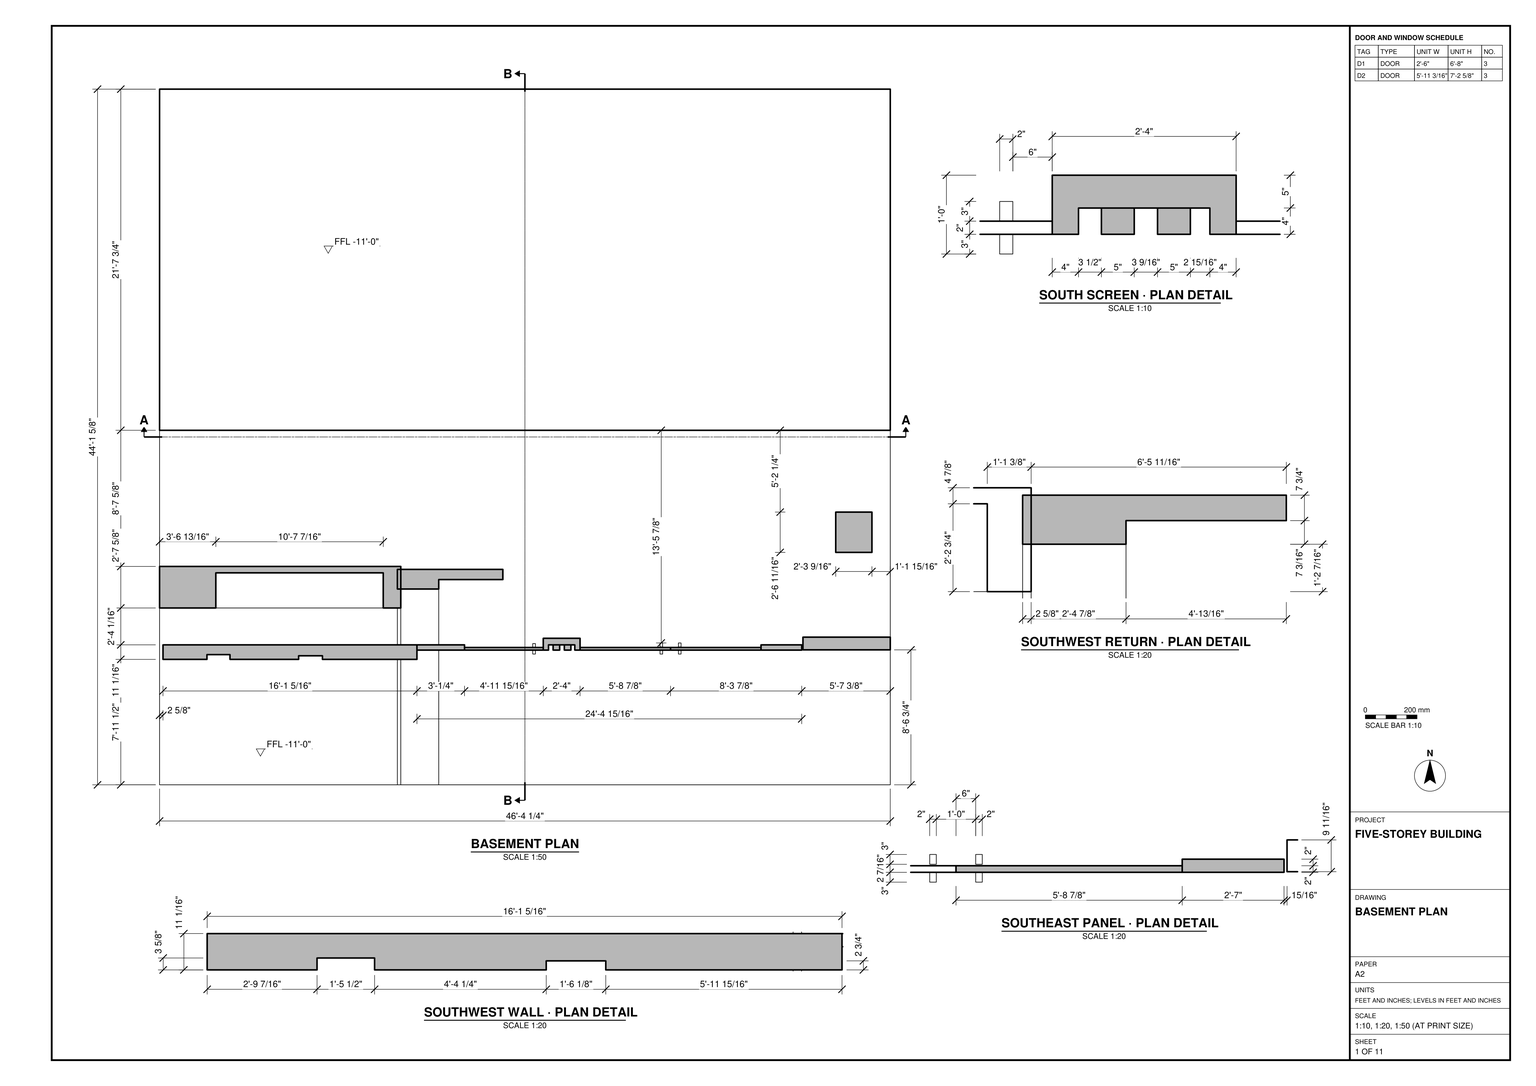
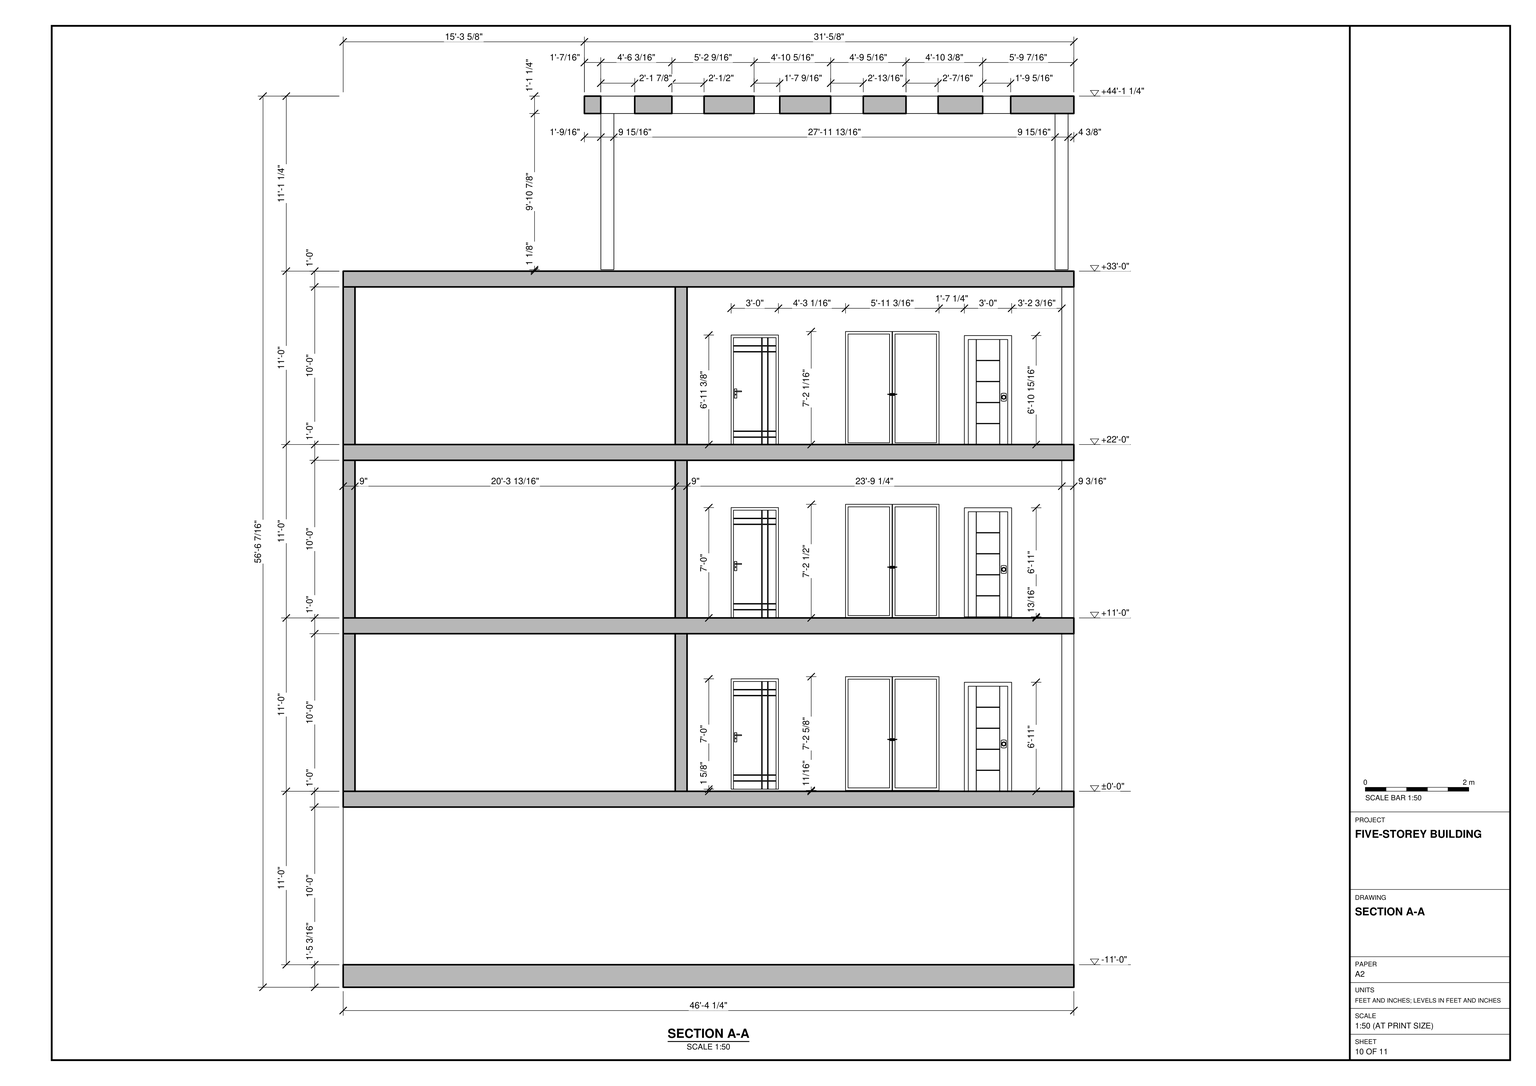
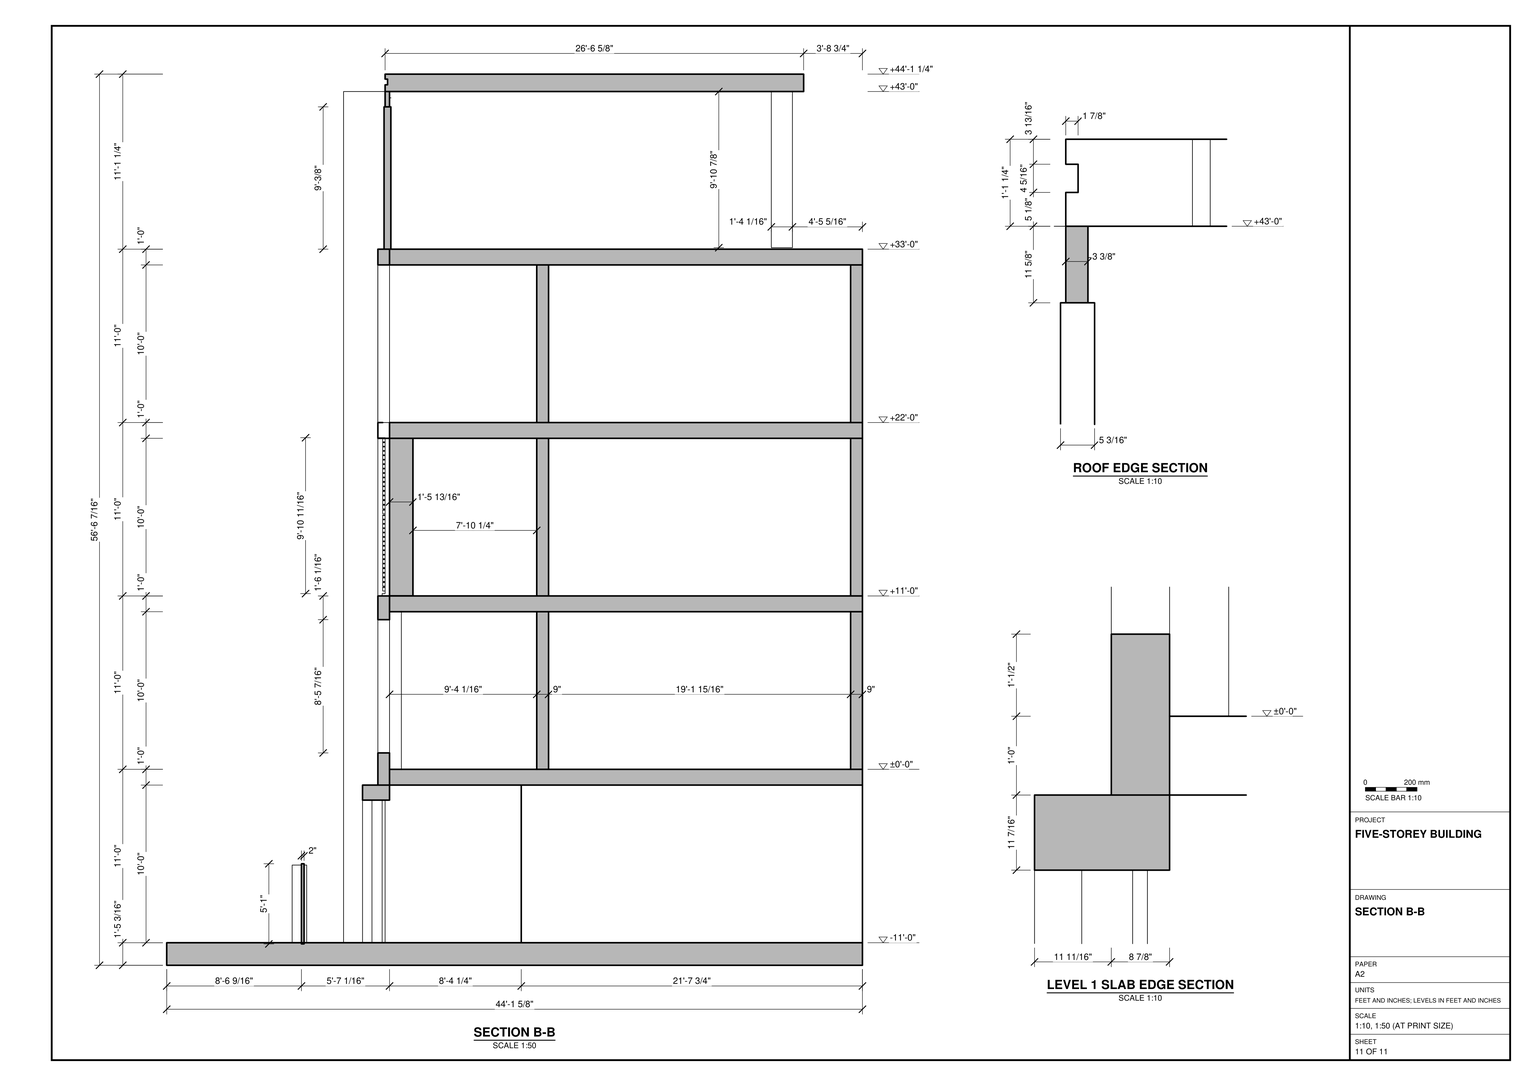
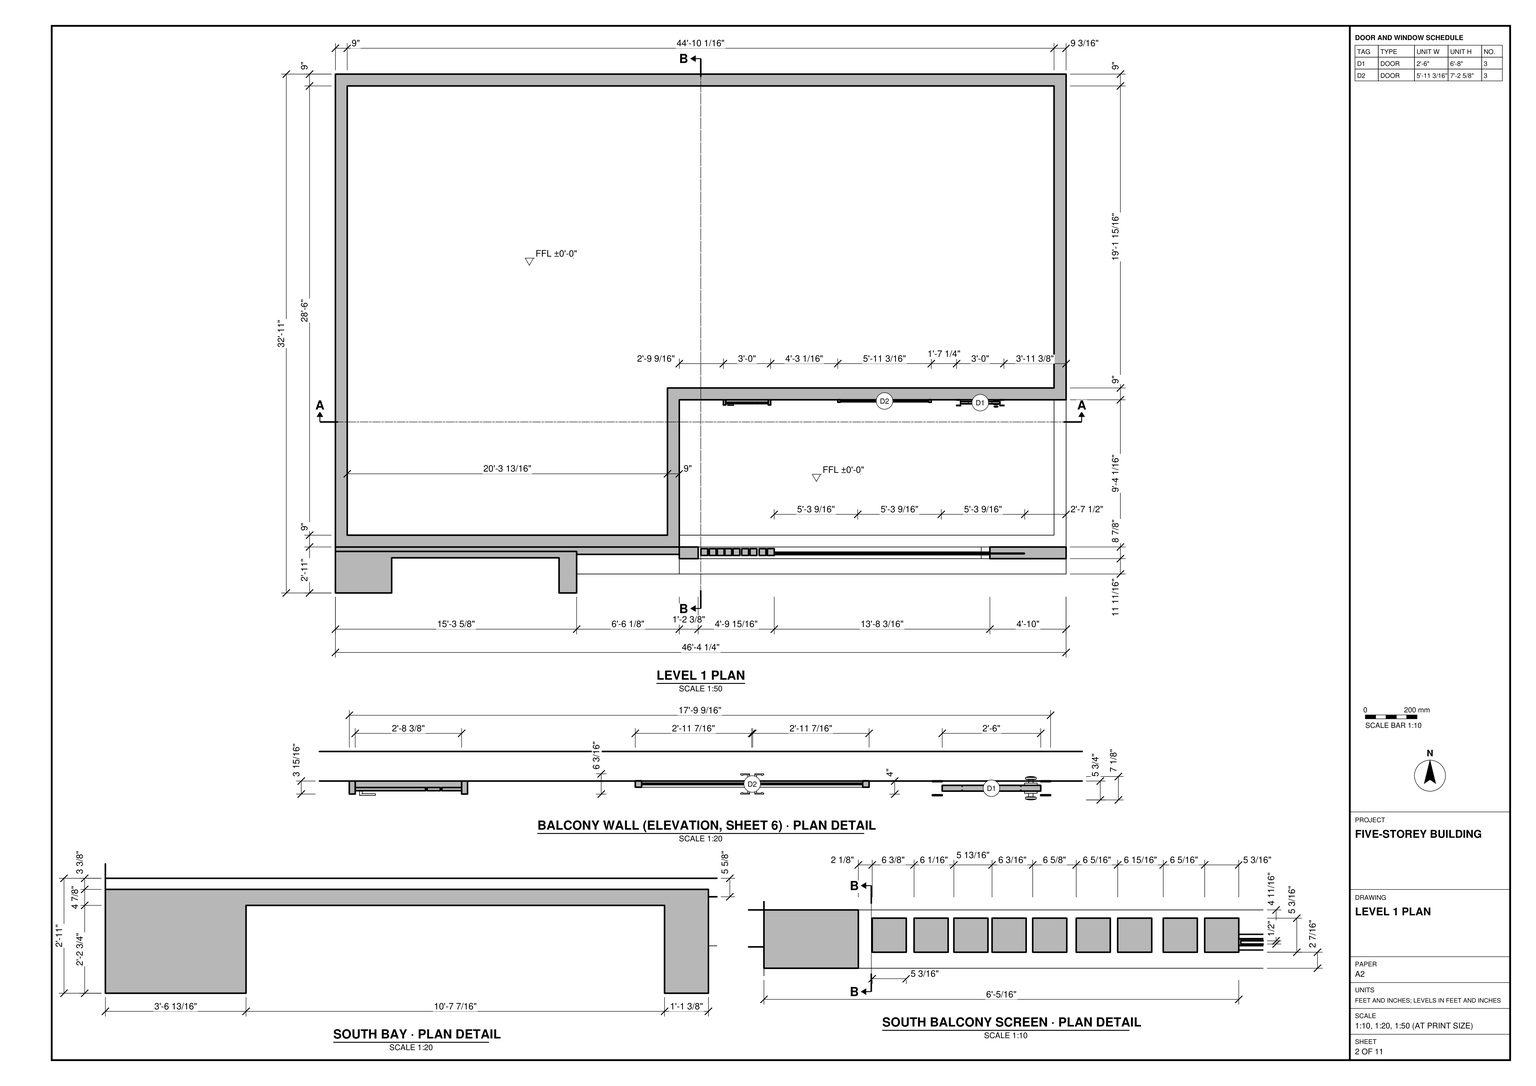
Build the building shown in task_files/diagram_01.pdf in SketchUp. Work in feet and inches. Orient the model with X east–west and Y north–south. The overall extents are 46'-4 1/4" along X, 44'-1 5/8" along Y and 56'-6 7/16" vertically. Set the basement at -11'-0", the ground floor at ±0'-0", and the remaining slab levels at +11'-0", +22'-0" and +33'-0".

Start with the basement slab, which extends south beyond the floors above. Use the enlarged basement plan details to shape the notched southwest wall, its return, the south screen and the southeast panel. Build the stacked floors with the wall thicknesses, slab edges and openings shown in the plans and sections. In section A-A, a pair of doors sits between two single doors; align this arrangement across the three floors shown. Use the plans to locate any stairs, built-in joinery and main furniture shown. Above the top slab, model the canopy supports and roof members, leaving the rest of the slab uncovered. Follow the roof edge section for the stepped profile.

Keep shell elements such as walls, slabs and roof separate as groups or components, and do the same for each furniture or joinery piece. Use components for repeated parts. Any decor and loose items shown may be suitable library components. Save one SketchUp model as output_files/five_storey_building_with_its_partial_rooftop_canopy.skp.

# SketchUp Ruby script. Lengths in inches.
U = 1.inch
M = Sketchup.active_model
def pt(a) = Geom::Point3d.new(a.map { |v| v * U })
def face(e, loops, mat)
  f = e.add_face(loops[0].map { |a| pt(a) })
  loops[1..].each { |l| e.add_face(l.map { |a| pt(a) }).erase! }
  f.material = f.back_material = mat if mat
  f
end
# faces: each face lists its corners as indices into pts; further lists are holes
def faces(e, pts, list, mat = nil) = list.each { |f| face(e, (f[0].is_a?(Array) ? f : [f]).map { |l| l.map { |i| pts[i] } }, mat) }
# xy, xz, yz: faces in a plane at the given z, y or x. An outline is a flat list of corners, or four numbers for a rectangle; further outlines are holes
def ring(l) = l.size == 4 ? [[l[0], l[1]], [l[2], l[1]], [l[2], l[3]], [l[0], l[3]]] : l.each_slice(2).to_a
def flat(e, list, mat, &to3) = list.each { |f| face(e, (f[0].is_a?(Array) ? f : [f]).map { |l| ring(l).map { |u, v| to3.(u, v) } }, mat) }
def xy(e, z, list, mat = nil) = flat(e, list, mat) { |x, y| [x, y, z] }
def xz(e, y, list, mat = nil) = flat(e, list, mat) { |x, z| [x, y, z] }
def yz(e, x, list, mat = nil) = flat(e, list, mat) { |y, z| [x, y, z] }
def lines(e, pts, list) = list.each { |a, b| e.add_line(pt(pts[a]), pt(pts[b])) }
# prism: a flat outline (further loops are holes) pulled along v
def prism(e, loops, v, mat = nil)
  f = face(e, loops, mat); d = Geom::Vector3d.new(v.map { |x| x * U })
  f.pushpull(f.normal.samedirection?(d) ? d.length : -d.length)
end
def box(e, o, s, mat = nil) = prism(e, [[o, [o[0] + s[0], o[1], o[2]], [o[0] + s[0], o[1] + s[1], o[2]], [o[0], o[1] + s[1], o[2]]]], [0, 0, s[2]], mat)
def at(x, y, z, deg = 0) = Geom::Transformation.translation(pt([x, y, z])) * Geom::Transformation.rotation(ORIGIN, Z_AXIS, deg.degrees)
def axes(o, x, y, z) = Geom::Transformation.new([*x, 0, *y, 0, *z, 0, *pt(o).to_a, 1])
def part(name) = M.definitions.add(name)
# library, detail: a bought-in or finely detailed component or shape, given as its bounding box
def library(name, o, s) = part(name).tap { |d| box(d.entities, o, s) }
def detail(e, o, s) = box(e.add_group.entities, o, s)
def put(e, d, t, mat = nil) = e.add_instance(d, t).tap { |i| i.material = mat if mat }
def group(e, t, mat = nil) = e.add_group.tap { |g| g.transformation = t; g.material = mat if mat }.entities
root = M.entities
M.materials.add("Glass_Window_Neutral\#2").color = [0, 0, 0]
M.materials["Glass_Window_Neutral\#2"].alpha = 0.125
M.materials.add("Iron_Blurry_5cm").color = [3, 3, 3]
M.materials.add("Material5, met").color = [196, 146, 107]
M.materials.add("[Color M00]").color = [255, 255, 255]
M.materials.add("[Color M09]").color = [0, 0, 0]
M.materials.add("[Granite Brown]").color = [126, 104, 91]
M.materials.add("[Granite Dark Gray]").color = [69, 68, 68]
M.materials.add("[Grass Dark Green]").color = [106, 157, 55]
M.materials.add("[Polished Concrete New]").color = [200, 200, 203]
M.materials.add("[Sandstone]").color = [118, 81, 52]
M.materials.add("[Stone Marble]").color = [214, 206, 203]
M.materials.add("[Translucent Glass Blue]").color = [100, 149, 237]
M.materials["[Translucent Glass Blue]"].alpha = 0.5
M.materials.add("polished steel").color = [183, 187, 190]
M.materials.add("polished, Blacktop Old 01").color = [132, 136, 139]
M.materials.add("steel").color = [179, 179, 179]
c1 = library("glass door",[0,0,0],[6.2,71.19,86.61])
c2 = library("Untitled (14)",[0,0,0],[7.13,36,83])
c3 = library("Untitled",[0,0,0],[36,4.39,84])
c4 = part("Framed glazing panel")
g1 = group(c4.entities,at(0,26.17,94.49),"[Color M09]")
xy(g1,-94.49,[[0,-26.17,1.18,0]],"Iron_Blurry_5cm")
xy(g1,-93.8,[[0,-25.51,0.59,-0.67],[0.59,-25.51,1.18,-0.67]],"Iron_Blurry_5cm")
xy(g1,-70.52,[[0.59,-25.51,1.18,-0.67]],"Iron_Blurry_5cm")
xy(g1,-69.84,[[0.59,-25.51,1.18,-0.67]],"Iron_Blurry_5cm")
xy(g1,-47.24,[[0.59,-25.51,1.18,-0.67]],"Iron_Blurry_5cm")
xy(g1,-46.56,[[0.59,-25.51,1.18,-0.67]],"Iron_Blurry_5cm")
xy(g1,-23.97,[[0.59,-25.51,1.18,-0.67]],"Iron_Blurry_5cm")
xy(g1,-23.28,[[0.59,-25.51,1.18,-0.67]],"Iron_Blurry_5cm")
xy(g1,-0.6875,[[0,-25.51,0.59,-0.67],[0.59,-25.51,1.18,-0.67]],"Iron_Blurry_5cm")
xy(g1,0,[[0,-26.17,1.18,0]],"Iron_Blurry_5cm")
xz(g1,-26.17,[[0,-94.49,1.18,0]],"Iron_Blurry_5cm")
xz(g1,-25.51,[[0,-93.8,0.59,-0.6875],[0.59,-93.8,1.18,-70.52],[0.59,-70.52,1.18,-69.84],[0.59,-69.84,1.18,-47.24],[0.59,-47.24,1.18,-46.56],
  [0.59,-46.56,1.18,-23.97],[0.59,-23.97,1.18,-23.28],[0.59,-23.28,1.18,-0.6875]],"Iron_Blurry_5cm")
xz(g1,-0.67,[[0,-93.8,0.59,-0.6875],[0.59,-93.8,1.18,-70.52],[0.59,-70.52,1.18,-69.84],[0.59,-69.84,1.18,-47.24],[0.59,-47.24,1.18,-46.56],
  [0.59,-46.56,1.18,-23.97],[0.59,-23.97,1.18,-23.28],[0.59,-23.28,1.18,-0.6875]],"Iron_Blurry_5cm")
xz(g1,0,[[0,-94.49,1.18,0]],"Iron_Blurry_5cm")
yz(g1,0,[[[-26.17,-94.49,0,0],[-25.51,-93.8,-0.67,-0.6875]]],"Iron_Blurry_5cm")
yz(g1,0.59,[[-25.51,-93.8,-0.67,-70.52],[-25.51,-69.84,-0.67,-47.24],[-25.51,-46.56,-0.67,-23.97],[-25.51,-23.28,-0.67,-0.6875]],"Glass_Window_Neutral\#2")
yz(g1,0.59,[[-25.51,-70.52,-0.67,-69.84],[-25.51,-47.24,-0.67,-46.56],[-25.51,-23.97,-0.67,-23.28]],"Iron_Blurry_5cm")
yz(g1,1.18,[[[-26.17,-94.49,0,0],[-25.51,-93.8,-0.67,-0.6875]],[-25.51,-70.52,-0.67,-69.84],[-25.51,-47.24,-0.67,-46.56],[-25.51,-23.97,-0.67,-23.28]],"Iron_Blurry_5cm")
g2 = group(c4.entities,at(0,52.35,94.49),"[Color M09]")
xy(g2,-94.49,[[0,-26.17,1.18,0]],"Iron_Blurry_5cm")
xy(g2,-93.8,[[0,-25.51,0.59,-0.67],[0.59,-25.51,1.18,-0.67]],"Iron_Blurry_5cm")
xy(g2,-70.52,[[0.59,-25.51,1.18,-0.67]],"Iron_Blurry_5cm")
xy(g2,-69.84,[[0.59,-25.51,1.18,-0.67]],"Iron_Blurry_5cm")
xy(g2,-47.24,[[0.59,-25.51,1.18,-0.67]],"Iron_Blurry_5cm")
xy(g2,-46.56,[[0.59,-25.51,1.18,-0.67]],"Iron_Blurry_5cm")
xy(g2,-23.97,[[0.59,-25.51,1.18,-0.67]],"Iron_Blurry_5cm")
xy(g2,-23.28,[[0.59,-25.51,1.18,-0.67]],"Iron_Blurry_5cm")
xy(g2,-0.6875,[[0,-25.51,0.59,-0.67],[0.59,-25.51,1.18,-0.67]],"Iron_Blurry_5cm")
xy(g2,0,[[0,-26.17,1.18,0]],"Iron_Blurry_5cm")
xz(g2,-26.17,[[0,-94.49,1.18,0]],"Iron_Blurry_5cm")
xz(g2,-25.51,[[0,-93.8,0.59,-0.6875],[0.59,-93.8,1.18,-70.52],[0.59,-70.52,1.18,-69.84],[0.59,-69.84,1.18,-47.24],[0.59,-47.24,1.18,-46.56],
  [0.59,-46.56,1.18,-23.97],[0.59,-23.97,1.18,-23.28],[0.59,-23.28,1.18,-0.6875]],"Iron_Blurry_5cm")
xz(g2,-0.67,[[0,-93.8,0.59,-0.6875],[0.59,-93.8,1.18,-70.52],[0.59,-70.52,1.18,-69.84],[0.59,-69.84,1.18,-47.24],[0.59,-47.24,1.18,-46.56],
  [0.59,-46.56,1.18,-23.97],[0.59,-23.97,1.18,-23.28],[0.59,-23.28,1.18,-0.6875]],"Iron_Blurry_5cm")
xz(g2,0,[[0,-94.49,1.18,0]],"Iron_Blurry_5cm")
yz(g2,0,[[[-26.17,-94.49,0,0],[-25.51,-93.8,-0.67,-0.6875]]],"Iron_Blurry_5cm")
yz(g2,0.59,[[-25.51,-93.8,-0.67,-70.52],[-25.51,-69.84,-0.67,-47.24],[-25.51,-46.56,-0.67,-23.97],[-25.51,-23.28,-0.67,-0.6875]],"Glass_Window_Neutral\#2")
yz(g2,0.59,[[-25.51,-70.52,-0.67,-69.84],[-25.51,-47.24,-0.67,-46.56],[-25.51,-23.97,-0.67,-23.28]],"Iron_Blurry_5cm")
yz(g2,1.18,[[[-26.17,-94.49,0,0],[-25.51,-93.8,-0.67,-0.6875]],[-25.51,-70.52,-0.67,-69.84],[-25.51,-47.24,-0.67,-46.56],[-25.51,-23.97,-0.67,-23.28]],"Iron_Blurry_5cm")
c5 = library("Wagner Glass Railing",[9.08,102.375,1.53],[2.51,145.5,42.05])
c6 = part("faewg")
xy(c6.entities,0,[[0,-3,2,0]])
xy(c6.entities,1,[[0,-2,2,0]])
xy(c6.entities,23,[[0,-2,2,0]])
xy(c6.entities,24,[[0,-3,2,0]])
xz(c6.entities,-3,[[0,0,2,24]],"polished steel")
xz(c6.entities,-2,[[0,1,2,23]])
xz(c6.entities,0,[[0,0,2,1],[0,23,2,24]])
yz(c6.entities,0,[[-3,0,-3,24,0,24,0,23,-2,23,-2,1,0,1,0,0]])
yz(c6.entities,2,[[-3,0,0,0,0,1,-2,1,-2,23,0,23,0,24,-3,24]])
c7 = part("reg")
xy(c7.entities,0,[[-8.95,3,59.93,5]])
xy(c7.entities,18,[[51.93,0,53.93,3]],"steel")
xy(c7.entities,19,[[51.93,1,53.93,3]],"steel")
xy(c7.entities,41,[[51.93,1,53.93,3]],"steel")
xy(c7.entities,42,[[51.93,0,53.93,3]],"steel")
xy(c7.entities,61,[[-8.95,3,59.93,5]])
xz(c7.entities,0,[[51.93,18,53.93,42]],"polished steel")
xz(c7.entities,1,[[51.93,19,53.93,41]],"steel")
xz(c7.entities,3,[[[-8.95,0,59.93,61],[51.93,18,53.93,19],[51.93,41,53.93,42]]])
xz(c7.entities,3,[[51.93,18,53.93,19],[51.93,41,53.93,42]],"steel")
xz(c7.entities,5,[[-8.95,0,59.93,61]])
yz(c7.entities,-8.95,[[3,0,5,61]])
yz(c7.entities,51.93,[[0,18,0,42,3,42,3,41,1,41,1,19,3,19,3,18]],"steel")
yz(c7.entities,53.93,[[0,18,3,18,3,19,1,19,1,41,3,41,3,42,0,42]],"steel")
yz(c7.entities,59.93,[[3,0,5,61]])
put(c7.entities,c6,axes([51.93,5.4375,42],[1,0,0],[0,-1,0],[0,0,-1]),"steel")
c8 = part("e3f")
xy(c8.entities,0,[[0,-2,59.93,0]])
xy(c8.entities,18,[[51.93,-5,53.93,-2]],"steel")
xy(c8.entities,19,[[51.93,-4,53.93,-2]],"steel")
xy(c8.entities,41,[[51.93,-4,53.93,-2]],"steel")
xy(c8.entities,42,[[51.93,-5,53.93,-2]],"steel")
xy(c8.entities,61,[[0,-2,59.93,0]])
xz(c8.entities,-5,[[51.93,18,53.93,42]],"polished steel")
xz(c8.entities,-4,[[51.93,19,53.93,41]],"steel")
xz(c8.entities,-2,[[[0,0,59.93,61],[51.93,41,53.93,42],[51.93,18,53.93,19]]])
xz(c8.entities,-2,[[51.93,18,53.93,19],[51.93,41,53.93,42]],"steel")
xz(c8.entities,0,[[0,0,59.93,61]])
yz(c8.entities,0,[[-2,0,0,61]])
yz(c8.entities,51.93,[[-5,18,-5,42,-2,42,-2,41,-4,41,-4,19,-2,19,-2,18]],"steel")
yz(c8.entities,53.93,[[-5,18,-2,18,-2,19,-4,19,-4,41,-2,41,-2,42,-5,42]],"steel")
yz(c8.entities,59.93,[[-2,0,0,61]])
put(c8.entities,c6,axes([51.93,0,42],[1,0,0],[0,-1,0],[0,0,-1]),"steel")
c9 = part("gbsrtn")
put(c9.entities,c7,at(402.95,-3,0))
put(c9.entities,c8,at(306.07,2,0))
put(c9.entities,c7,axes([522.82,-3,0],[-1,0,0],[0,1,0],[0,0,1]))
g3 = group(c9.entities,at(366,9,0),"polished, Blacktop Old 01")
xy(g3,0,[[0,-9,0,0,28,0,28,-9,24,-9,24,-5,4,-5,4,-9]])
xy(g3,60,[[0,-9,4,-9,4,-5,24,-5,24,-9,28,-9,28,0,0,0]],"[Polished Concrete New]")
xz(g3,-9,[[0,0,4,60],[24,0,28,60]],"[Polished Concrete New]")
xz(g3,-5,[[4,0,24,60]],"Material5, met")
xz(g3,0,[[0,0,28,60]])
yz(g3,0,[[-9,0,0,60]],"[Polished Concrete New]")
yz(g3,4,[[-9,0,-5,60]],"polished, Blacktop Old 01")
yz(g3,24,[[-9,0,-5,60]],"polished, Blacktop Old 01")
yz(g3,28,[[-9,0,0,60]],"[Polished Concrete New]")
g4 = group(c9.entities,at(12.5,0,0))
prism(g4,[[[365.99,4,0],[365.99,4,4],[365.99,4,56],[365.99,4,60],[365.99,0,60],[365.99,0,0]]],[-5,0,0])
prism(g4,[[[374.53,4,0],[374.53,4,4],[374.53,4,56],[374.53,4,60],[374.53,0,60],[374.53,0,0]]],[-5,0,0])
g5 = group(c9.entities,at(29.55,0,0))
box(g5,[502.22,0,0],[31,4,60],"[Polished Concrete New]")
box(g5,[240.29,0,0],[36.23,4,60],"[Polished Concrete New]")
c10 = part("main gate")
put(c10.entities,c9,at(-149.07,478.25,-161.76),"[Grass Dark Green]")
c11 = part("Group\#1")
box(c11.entities,[0,-360,0],[556.25,360,12])
c12 = part("Group\#9")
box(c12.entities,[0,0,0],[5.1875,5.1875,132])
c13 = part("Group\#3")
box(c13.entities,[0,0,0],[5.1875,5.1875,101.4375])
c14 = part("Group\#5")
box(c14.entities,[0,0,0],[5.0625,5.0625,87.3125])
c15 = part("Group\#7")
prism(c15.entities,[[[0,0,0],[0,0,3.13],[78.15,0,3.13],[78.15,0,2.68],[78.15,0,0]]],[0,-1.8125,0])
prism(c15.entities,[[[0,0,-3.3125],[0,0,-0.18],[78.15,0,-0.18],[78.15,0,-0.64],[78.15,0,-3.3125]]],[0,-1.8125,0])
prism(c15.entities,[[[0,-1.8125,-3.49],[0,-1.8125,-6.625],[78.15,-1.8125,-6.625],[78.15,-1.8125,-3.95],[78.15,-1.8125,-3.49]]],[0,1.8125,0])
prism(c15.entities,[[[0,0,-9.875],[0,0,-6.74],[78.15,0,-6.74],[78.15,0,-7.2],[78.15,0,-9.875]]],[0,-1.8125,0])
prism(c15.entities,[[[0,0,-13.25],[0,0,-10.12],[78.15,0,-10.12],[78.15,0,-10.57],[78.15,0,-13.25]]],[0,-1.8125,0])
prism(c15.entities,[[[0,-1.8125,-13.49],[0,-1.8125,-16.625],[78.15,-1.8125,-16.625],[78.15,-1.8125,-13.95],[78.15,-1.8125,-13.49]]],[0,1.8125,0])
prism(c15.entities,[[[0,0,-20],[0,0,-16.87],[78.15,0,-16.87],[78.15,0,-17.32],[78.15,0,-20]]],[0,-1.8125,0])
prism(c15.entities,[[[0,0,-23.375],[0,0,-20.24],[78.15,0,-20.24],[78.15,0,-20.7],[78.15,0,-23.375]]],[0,-1.8125,0])
prism(c15.entities,[[[0,-1.8125,-23.62],[0,-1.8125,-26.75],[78.15,-1.8125,-26.75],[78.15,-1.8125,-24.07],[78.15,-1.8125,-23.62]]],[0,1.8125,0])
prism(c15.entities,[[[0,0,-30.125],[0,0,-26.99],[78.15,0,-26.99],[78.15,0,-27.45],[78.15,0,-30.125]]],[0,-1.8125,0])
prism(c15.entities,[[[0,-1.8125,-30.43],[0,-1.8125,-33.5625],[78.15,-1.8125,-33.5625],[78.15,-1.8125,-30.89],[78.15,-1.8125,-30.43]]],[0,1.8125,0])
prism(c15.entities,[[[0,-1.8125,-33.74],[0,-1.8125,-36.875],[78.15,-1.8125,-36.875],[78.15,-1.8125,-34.2],[78.15,-1.8125,-33.74]]],[0,1.8125,0])
prism(c15.entities,[[[0,-1.8125,-37.31],[0,-1.8125,-40.4375],[78.15,-1.8125,-40.4375],[78.15,-1.8125,-37.76],[78.15,-1.8125,-37.31]]],[0,1.8125,0])
prism(c15.entities,[[[0,-1.8125,-40.74],[0,-1.8125,-43.875],[78.15,-1.8125,-43.875],[78.15,-1.8125,-41.2],[78.15,-1.8125,-40.74]]],[0,1.8125,0])
prism(c15.entities,[[[0,-1.8125,-44.37],[0,-1.8125,-47.5],[78.15,-1.8125,-47.5],[78.15,-1.8125,-44.82],[78.15,-1.8125,-44.37]]],[0,1.8125,0])
prism(c15.entities,[[[0,-1.8125,-47.87],[0,-1.8125,-51],[78.15,-1.8125,-51],[78.15,-1.8125,-48.32],[78.15,-1.8125,-47.87]]],[0,1.8125,0])
prism(c15.entities,[[[0,0,-54.75],[0,0,-51.62],[78.15,0,-51.62],[78.15,0,-52.07],[78.15,0,-54.75]]],[0,-1.8125,0])
c16 = part("Group\#8")
box(c16.entities,[0,-0.6875,0],[69.3,0.6875,3.73])
c17 = part("Group\#4")
box(c17.entities,[0,0,0],[5.1875,5.1875,108.35])
c18 = part("Group\#10")
box(c18.entities,[0,0,0],[9.9375,16.08,118.875])
xy(root,-149.1875,[[0,0,556.25,529.625]])
xy(root,-132,[[0,0,181.03,0,181.03,95.49,124,95.49,124,98.24,105.86,98.24,105.86,95.49,53.6,95.49,53.6,99.12,36.07,99.12,36.07,95.49,2.61,95.49,2.61,106.55,181.03,106.55,181.03,134.625,0,134.625],[212.51,0,556.25,0,556.25,102.74,489.78,102.74,489.78,112.42,556.25,112.42,556.25,269.9,0,269.9,0,166.25,183.63,166.25,183.63,164,261.33,164,261.33,156.25,212.51,156.25],[181.03,0,183.63,95.49],[183.63,0,212.51,0,212.51,149.0625,183.63,149.0625,183.63,106.55,195.93,106.55,195.93,95.49,183.63,95.49],[181.03,106.55,183.63,134.625],
  [0,134.625,0,166.25,183.63,166.25,183.63,164,181.03,164,181.03,134.625],[181.03,134.625,183.63,149.0625],[181.03,149.0625,183.63,164],[183.63,149.0625,212.51,164],[212.51,156.25,261.33,164],
  [212.51,156.25,261.33,164],[0,269.9,556.25,529.625]])
xy(root,-117.02,[[42.83,134.625,170.27,161.375]])
xy(root,-72.89,[[2.61,95.49,36.07,95.49,36.07,99.12,53.6,99.12,53.6,95.49,105.86,95.49,105.86,98.24,124,98.24,124,95.49,195.93,95.49,195.93,106.55,2.61,106.55],[489.78,102.74,556.25,112.42]])
xy(root,-23.4375,[[212.51,149.0625,212.51,156.25,261.33,156.25,261.33,164,261.78,164,261.78,169.625,556.25,169.625,556.25,149.0625]])
xy(root,-12,[[181.03,149.0625,261.78,164],[261.78,149.0625,556.25,160.75],[261.78,160.75,556.25,169.625],[183.63,164,183.63,166.25,0,166.25,0,169.625,261.78,169.625,261.78,164],[0,269.9,556.25,529.625]])
xy(root,0,[[[0,169.625,261.78,169.625,261.78,281.6875,556.25,281.6875,556.25,529.625,0,529.625],[9,178.625,9,520.625,547.0625,520.625,547.0625,290.6875,252.78,290.6875,252.78,178.625]],[261.78,169.625,556.25,169.625,556.25,281.6875,547.0625,281.6875,547.0625,178.625,261.78,178.625],[9,178.625,252.78,178.625,252.78,290.6875,547.0625,290.6875,547.0625,520.625,9,520.625]])
xy(root,0,[[261.78,178.625,547.0625,281.6875]],"[Color M00]")
xy(root,12.5,[[276.15,160.75,491.63,169.625]])
xy(root,74.73,[[74.54,149.875,144.61,161.375]],"[Stone Marble]")
xy(root,82.84,[[82.66,149.875,136.49,161.375]],"[Stone Marble]")
xy(root,113.9375,[[276.15,160.75,488.01,169.625],[488.01,160.75,498.24,169.625]])
xy(root,120,[[[0,169.625,261.78,169.625,261.78,281.6875,556.25,281.6875,556.25,529.625,0,529.625],[9,178.625,9,520.625,547.0625,520.625,547.0625,290.6875,252.78,290.6875,252.78,178.625]]])
xy(root,132,[[261.78,160.75,556.25,169.625],[[0,169.625,261.78,169.625,261.78,281.6875,556.25,281.6875,556.25,529.625,0,529.625],[9,178.625,9,520.625,547.0625,520.625,547.0625,290.6875,252.78,290.6875,252.78,178.625]],[261.78,169.625,556.25,169.625,556.25,281.6875,547.0625,281.6875,547.0625,178.625,261.78,178.625],[9,178.625,252.78,178.625,252.78,290.6875,547.0625,290.6875,547.0625,520.625,9,520.625]])
xy(root,132.0625,[[519.2,160.75,556.25,170.3125],[261.78,169.625,261.78,187.4375,556.25,187.4375,556.25,170.3125,519.2,170.3125,519.2,169.625]])
xy(root,133.78,[[183.63,164,261.78,166.25]])
xy(root,152.84,[[329.09,169.625,500.01,187.4375]])
xy(root,234.78,[[329.91,169.625,500.01,187.4375]])
xy(root,252,[[261.78,160.75,519.2,169.625],[519.2,160.75,556.25,169.625],[[0,169.625,261.78,169.625,261.78,281.6875,556.25,281.6875,556.25,529.625,0,529.625],[9,178.625,9,520.625,547.0625,520.625,547.0625,290.6875,252.78,290.6875,252.78,178.625]],[519.2,169.625,556.25,170.3125]])
xy(root,252.46,[[183.63,160.6875,261.78,166.25]],"[Granite Dark Gray]")
xy(root,264,[[276.15,160.75,481.8,160.75,481.8,169.625,283.3125,169.625,283.3125,164.4375,278.125,164.4375,278.125,169.625,276.15,169.625],[[0,169.625,261.78,169.625,261.78,281.6875,556.25,281.6875,556.25,529.625,0,529.625],[9,178.625,9,520.625,547.0625,520.625,547.0625,290.6875,252.78,290.6875,252.78,178.625]],[481.8,169.625,498.24,169.9375],[9,178.625,252.78,178.625,252.78,290.6875,547.0625,290.6875,547.0625,520.625,9,520.625]])
xy(root,384,[[276.15,160.75,477.47,169.625],[[0,169.625,261.78,169.625,261.78,281.6875,556.25,281.6875,556.25,529.625,0,529.625],[9,178.625,9,520.625,547.0625,520.625,547.0625,290.6875,252.78,290.6875,252.78,178.625]]])
xy(root,388.11,[[82.66,149.875,136.49,161.375]],"[Stone Marble]")
xy(root,396,[[261.78,160.75,556.25,169.625],[0,166.25,183.63,169.625]])
xy(root,396,[[183.63,160.6875,192.48,166.25],[192.48,160.6875,261.78,167.9375]],"[Granite Dark Gray]")
xy(root,396.23,[[74.54,149.875,144.61,161.375]],"[Stone Marble]")
xy(root,497.48,[[42.83,134.625,170.27,161.375]])
xy(root,504.35,[[192.48,166.25,192.48,167.9375,261.78,167.9375,261.78,169.625,334.375,169.625,334.375,166.25]])
xy(root,516,[[0,134.625,183.63,166.25],[183.63,166.25,334.375,169.625],[[334.375,166.25,334.375,169.625,183.63,169.625,183.63,484.875,556.25,484.875,556.25,166.25],[196.08,185.54,221.96,460.1],[371.12,188.73,395.93,470.35],[428.46,191.91,452.9,473.28],[250.24,188.24,274.74,461.05],[486.84,192.91,508.15,473.97],[312.8125,190.07,332.375,467.51]]])
xy(root,521.15,[[183.63,166.25,556.25,168.125]])
xy(root,525.44,[[183.63,166.25,556.25,168.125]])
xy(root,529.25,[[[183.63,166.25,556.25,484.875],[196.08,185.54,221.96,460.1],[371.12,188.73,395.93,470.35],[428.46,191.91,452.9,473.28],[250.24,188.24,274.74,461.05],[486.84,192.91,508.15,473.97],[312.8125,190.07,332.375,467.51]]])
xz(root,0,[[0,-149.1875,556.25,-132]])
xz(root,95.49,[[2.61,-132,36.07,-72.89],[53.6,-132,105.86,-72.89],[124,-132,195.93,-106.4],[124,-106.4,195.93,-72.89]])
xz(root,98.24,[[105.86,-132,124,-72.89]],"[Sandstone]")
xz(root,99.12,[[36.07,-132,53.6,-72.89]],"[Sandstone]")
xz(root,102.74,[[489.78,-132,556.25,-72.89]])
xz(root,106.55,[[2.61,-132,195.93,-72.89]])
xz(root,112.42,[[489.78,-132,556.25,-72.89]])
xz(root,134.625,[[[0,-132,183.63,516],[42.83,-117.02,170.27,497.48]]])
xz(root,149.0625,[[181.03,-132,212.51,-132,212.51,-23.4375,556.25,-23.4375,556.25,-12,181.03,-12]])
xz(root,149.875,[[[74.54,74.73,144.61,396.23],[82.66,82.84,136.49,388.11]]],"[Stone Marble]")
xz(root,156.25,[[212.51,-132,261.33,-23.4375]])
xz(root,160.6875,[[183.63,252.46,261.78,396]],"[Granite Dark Gray]")
xz(root,160.75,[[[261.78,-12,556.25,132],[276.15,12.5,276.15,113.9375,488.01,113.9375,489.25,113.625,490.45,113.19,491.61,112.64,492.7,111.99,493.72,111.23,494.67,110.37,495.53,109.42,496.29,108.4,496.95,107.3,497.49,106.15,497.93,104.95,498.24,103.71,498.24,19.11,498.18,18.25,498.01,17.4,497.74,16.58,497.35,15.8,496.875,15.09,496.3,14.4375,495.65,13.87,494.94,13.39,494.16,13,493.34,12.73,492.49,12.56,491.63,12.5]],[[261.78,252,556.25,396],[276.15,264,276.15,384,477.47,384,480.375,383.04,483.16,381.77,485.79,380.21,488.23,378.37,490.46,376.27,492.45,373.94,494.18,371.42,495.62,368.72,496.75,365.875,497.58,362.93,498.07,359.91,498.24,356.85,498.24,278.01,497.82,276.09,497.17,274.25,496.3125,272.49,495.26,270.84,494.01,269.33,492.6,267.98,491.04,266.8,489.35,265.81,487.55,265.03,485.68,264.46,483.75,264.12,481.8,264]]])
xz(root,160.75,[[519.2,132.0625,556.25,252]],"[Granite Brown]")
xz(root,161.375,[[[42.83,-117.02,170.27,497.48],[74.54,74.73,144.61,396.23]],[82.66,82.84,136.49,388.11]],"[Stone Marble]")
xz(root,164,[[181.03,-132,183.63,-12],[183.63,-132,183.63,-12,261.78,-12,261.78,-23.4375,261.33,-23.4375,261.33,-132]])
xz(root,164,[[183.63,-12,261.78,133.78]],"[Granite Dark Gray]")
xz(root,166.25,[[0,-132,183.63,-12],[0,-12,183.63,396],[183.63,133.78,261.78,249.32],[0,396,183.63,516],[183.63,396,192.48,396,192.48,504.35,334.375,504.35,334.375,516,183.63,516],
  [183.63,516,556.25,521.15],[183.63,525.44,556.25,529.25]])
xz(root,167.9375,[[192.48,396,261.78,500.62]])
xz(root,168.125,[[183.63,521.15,556.25,525.44]])
xz(root,169.625,[[261.78,-23.4375,556.25,-12],[0,-12,261.78,0],[261.78,-12,556.25,0],[0,0,261.78,120],[261.78,0,498.24,12.5],
  [498.24,0,498.24,113.9375,276.15,113.9375,276.15,12.5,261.78,12.5,261.78,132,556.25,132,556.25,0],[491.63,12.5,492.49,12.56,493.34,12.73,494.16,13,494.94,13.39,495.65,13.87,496.3,14.4375,496.875,15.09,497.35,15.8,497.74,16.58,498.01,17.4,498.18,18.25,498.24,19.11,498.24,12.5],[498.24,103.71,497.93,104.95,497.49,106.15,496.95,107.3,496.29,108.4,495.53,109.42,494.67,110.37,493.72,111.23,492.7,111.99,491.61,112.64,490.45,113.19,489.25,113.625,488.01,113.9375,498.24,113.9375],[0,120,261.78,132],[0,132,261.78,252],
  [[261.78,132.0625,519.2,252],[329.09,152.84,326.75,152.99,324.44,153.45,322.22,154.21,320.11,155.25,318.16,156.55,316.4,158.1,314.85,159.87,313.54,161.82,312.5,163.92,311.75,166.15,311.29,168.45,311.14,170.79,311.14,216,311.3,218.45,311.78,220.86,312.57,223.1875,313.65,225.39,315.02,227.43,316.64,229.28,318.48,230.9,320.53,232.26,322.73,233.35,325.05,234.14,327.46,234.62,329.91,234.78,500.01,234.78,500.01,152.84]],[0,252,261.78,264],[261.78,252,556.25,264],[0,264,261.78,384],[261.78,264,261.78,396,556.25,396,556.25,384,276.15,384,276.15,264],
  [498.24,264,556.25,384],[498.24,356.85,498.07,359.91,497.58,362.93,496.75,365.875,495.62,368.72,494.18,371.42,492.45,373.94,490.46,376.27,488.23,378.37,485.79,380.21,483.16,381.77,480.375,383.04,477.47,384,498.24,384],[0,384,0,396,183.63,396,183.63,516,334.375,516,334.375,504.35,261.78,504.35,261.78,384]])
xz(root,169.9375,[[481.8,264,483.75,264.12,485.68,264.46,487.55,265.03,489.35,265.81,491.04,266.8,492.6,267.98,494.01,269.33,495.26,270.84,496.3125,272.49,497.17,274.25,497.82,276.09,498.24,278.01,498.24,264]])
xz(root,170.3125,[[519.2,132.0625,556.25,252]])
xz(root,178.625,[[9,0,252.78,120],[9,132,252.78,252],[9,264,252.78,384]])
xz(root,185.54,[[196.08,516,221.96,529.25]])
xz(root,187.4375,[[[261.78,132.0625,556.25,252],[311.14,152.84,500.01,234.78]]])
xz(root,188.24,[[250.24,516,274.74,529.25]])
xz(root,188.73,[[371.12,516,395.93,529.25]])
xz(root,190.07,[[312.8125,516,332.375,529.25]])
xz(root,191.91,[[428.46,516,452.9,529.25]])
xz(root,192.91,[[486.84,516,508.15,529.25]])
xz(root,269.9,[[0,-132,556.25,-12]],"[Sandstone]")
xz(root,281.6875,[[261.78,0,547.0625,120],[547.0625,0,556.25,120],[261.78,132,547.0625,252],[547.0625,132,556.25,252],[261.78,264,547.0625,384],
  [547.0625,264,556.25,384]])
xz(root,290.6875,[[252.78,0,547.0625,120],[252.78,132,547.0625,252],[252.78,264,547.0625,384]])
xz(root,460.1,[[196.08,516,221.96,529.25]])
xz(root,461.05,[[250.24,516,274.74,529.25]])
xz(root,467.51,[[312.8125,516,332.375,529.25]])
xz(root,470.35,[[371.12,516,395.93,529.25]])
xz(root,473.28,[[428.46,516,452.9,529.25]])
xz(root,473.97,[[486.84,516,508.15,529.25]])
xz(root,484.875,[[183.63,516,556.25,529.25]])
xz(root,520.625,[[9,0,547.0625,120],[9,132,547.0625,252],[9,264,547.0625,384]])
xz(root,529.625,[[0,-149.1875,556.25,-132],[0,-132,556.25,-12],[0,0,556.25,120],[0,132,556.25,252],[0,264,556.25,384]])
yz(root,0,[[0,-149.1875,529.625,-132],[134.625,-132,166.25,516],[269.9,-132,529.625,-12],[166.25,-12,169.625,396],[169.625,0,529.625,120],
  [169.625,132,529.625,252],[169.625,264,529.625,384]])
yz(root,2.61,[[95.49,-132,106.55,-72.89]])
yz(root,9,[[178.625,0,520.625,120],[178.625,132,520.625,252],[178.625,264,520.625,384]])
yz(root,36.07,[[95.49,-132,99.12,-72.89]])
yz(root,42.83,[[134.625,-117.02,161.375,497.48]])
yz(root,53.6,[[95.49,-132,99.12,-72.89]])
yz(root,74.54,[[149.875,74.73,161.375,396.23]],"[Stone Marble]")
yz(root,82.66,[[149.875,82.84,161.375,388.11]],"[Stone Marble]")
yz(root,105.86,[[95.49,-132,98.24,-72.89]])
yz(root,124,[[95.49,-132,98.24,-72.89]])
yz(root,136.49,[[149.875,82.84,161.375,388.11]],"[Stone Marble]")
yz(root,144.61,[[149.875,74.73,161.375,396.23]],"[Stone Marble]")
yz(root,170.27,[[134.625,-117.02,161.375,497.48]])
yz(root,181.03,[[149.0625,-132,164,-12]])
yz(root,183.63,[[134.625,-132,164,-132,164,133.78,166.25,133.78,166.25,252.46,160.6875,252.46,160.6875,396,166.25,396,166.25,516,134.625,516],[164,-132,166.25,-12],[164,-12,166.25,133.78],[160.6875,252.46,166.25,396],[166.25,396,169.625,516],
  [166.25,516,166.25,521.15,168.125,521.15,168.125,525.44,166.25,525.44,166.25,529.25,484.875,529.25,484.875,516]])
yz(root,192.48,[[166.25,396,167.9375,504.35]])
yz(root,195.93,[[95.49,-132,106.55,-72.89]])
yz(root,196.08,[[185.54,516,460.1,529.25]])
yz(root,212.51,[[149.0625,-132,156.25,-23.4375]])
yz(root,221.96,[[185.54,516,460.1,529.25]])
yz(root,250.24,[[188.24,516,461.05,529.25]])
yz(root,252.78,[[178.625,0,290.6875,120],[178.625,132,290.6875,252],[178.625,264,290.6875,384]])
yz(root,261.33,[[156.25,-132,164,-23.4375]])
yz(root,261.78,[[164,-23.4375,169.625,-12],[160.75,-12,164,12.5],[164,-12,169.625,12.5],[169.625,0,178.625,120],[178.625,0,281.6875,120],
  [160.75,12.5,164,132],[164,12.5,169.625,132],[160.75,132,160.75,252,166.25,252,166.25,133.78,164,133.78,164,132],[164,132,164,133.78,166.25,133.78,166.25,252,169.625,252,169.625,132],[169.625,132,178.625,132.0625],
  [178.625,132,281.6875,132,281.6875,252,187.4375,252,187.4375,132.0625,178.625,132.0625],[169.625,132.0625,178.625,252],[178.625,132.0625,187.4375,252],[160.75,252,166.25,252.46],[166.25,252,169.625,252,169.625,396,160.75,396,160.75,252.46,166.25,252.46],
  [160.6875,252.46,160.75,396],[169.625,264,281.6875,384],[167.9375,396,169.625,504.35]])
yz(root,274.74,[[188.24,516,461.05,529.25]])
yz(root,276.15,[[160.75,12.5,169.625,113.9375],[160.75,264,169.625,384]])
yz(root,311.14,[[169.625,170.79,187.4375,216]])
yz(root,312.8125,[[190.07,516,467.51,529.25]])
yz(root,332.375,[[190.07,516,467.51,529.25]])
yz(root,334.375,[[166.25,504.35,169.625,516]])
yz(root,371.12,[[188.73,516,470.35,529.25]])
yz(root,395.93,[[188.73,516,470.35,529.25]])
yz(root,428.46,[[191.91,516,473.28,529.25]])
yz(root,452.9,[[191.91,516,473.28,529.25]])
yz(root,486.84,[[192.91,516,473.97,529.25]])
yz(root,489.78,[[102.74,-132,112.42,-72.89]])
yz(root,498.24,[[160.75,19.11,169.625,103.71],[169.625,264,169.9375,278.01],[160.75,278.01,169.625,356.85]])
yz(root,500.01,[[169.625,152.84,187.4375,234.78]])
yz(root,508.15,[[192.91,516,473.97,529.25]])
yz(root,519.2,[[160.75,132.0625,169.625,252],[169.625,132.0625,170.3125,252]])
yz(root,547.0625,[[290.6875,0,520.625,120],[290.6875,132,520.625,252],[290.6875,264,520.625,384]])
yz(root,556.25,[[0,-149.1875,529.625,-149.1875,529.625,-132,112.42,-132,112.42,-72.89,102.74,-72.89,102.74,-132,0,-132],[269.9,-132,529.625,-12],[149.0625,-23.4375,169.625,-12],[160.75,-12,169.625,132],[281.6875,0,529.625,120],
  [281.6875,132,529.625,252],[160.75,132.0625,170.3125,252],[170.3125,132.0625,187.4375,252],[160.75,252,169.625,384],[281.6875,264,529.625,384],
  [160.75,384,169.625,396],[166.25,516,484.875,516,484.875,529.25,166.25,529.25,166.25,525.44,168.125,525.44,168.125,521.15,166.25,521.15]])
p = [[491.63,160.75,12.5],[492.49,160.75,12.56],[492.49,169.625,12.56],[491.63,169.625,12.5],[493.34,160.75,12.73],[493.34,169.625,12.73],
  [494.16,160.75,13],[494.16,169.625,13],[494.94,160.75,13.39],[494.94,169.625,13.39],[495.65,160.75,13.87],[495.65,169.625,13.87],
  [496.3,160.75,14.4375],[496.3,169.625,14.4375],[496.875,160.75,15.09],[496.875,169.625,15.09],[497.35,160.75,15.8],[497.35,169.625,15.8],
  [497.74,160.75,16.58],[497.74,169.625,16.58],[498.01,160.75,17.4],[498.01,169.625,17.4],[498.18,160.75,18.25],[498.18,169.625,18.25],
  [498.24,160.75,19.11],[498.24,169.625,19.11],[498.24,160.75,103.71],[497.93,160.75,104.95],[497.93,169.625,104.95],[498.24,169.625,103.71],
  [497.49,160.75,106.15],[497.49,169.625,106.15],[496.95,160.75,107.3],[496.95,169.625,107.3],[496.29,160.75,108.4],[496.29,169.625,108.4],
  [495.53,160.75,109.42],[495.53,169.625,109.42],[494.67,160.75,110.37],[494.67,169.625,110.37],[493.72,160.75,111.23],[493.72,169.625,111.23],
  [492.7,160.75,111.99],[492.7,169.625,111.99],[491.61,160.75,112.64],[491.61,169.625,112.64],[490.45,160.75,113.19],[490.45,169.625,113.19],
  [489.25,160.75,113.625],[489.25,169.625,113.625],[488.01,160.75,113.9375],[488.01,169.625,113.9375],[326.75,169.625,152.99],[329.09,169.625,152.84],
  [329.09,187.4375,152.84],[326.75,187.4375,152.99],[324.44,169.625,153.45],[324.44,187.4375,153.45],[322.22,169.625,154.21],[322.22,187.4375,154.21],
  [320.11,169.625,155.25],[320.11,187.4375,155.25],[318.16,169.625,156.55],[318.16,187.4375,156.55],[316.4,169.625,158.1],[316.4,187.4375,158.1],
  [314.85,169.625,159.87],[314.85,187.4375,159.87],[313.54,169.625,161.82],[313.54,187.4375,161.82],[312.5,169.625,163.92],[312.5,187.4375,163.92],
  [311.75,169.625,166.15],[311.75,187.4375,166.15],[311.29,169.625,168.45],[311.29,187.4375,168.45],[311.14,169.625,170.79],[311.14,187.4375,170.79],
  [311.3,169.625,218.45],[311.14,169.625,216],[311.14,187.4375,216],[311.3,187.4375,218.45],[311.78,169.625,220.86],[311.78,187.4375,220.86],
  [312.57,169.625,223.1875],[312.57,187.4375,223.1875],[313.65,169.625,225.39],[313.65,187.4375,225.39],[315.02,169.625,227.43],[315.02,187.4375,227.43],
  [316.64,169.625,229.28],[316.64,187.4375,229.28],[318.48,169.625,230.9],[318.48,187.4375,230.9],[320.53,169.625,232.26],[320.53,187.4375,232.26],
  [322.73,169.625,233.35],[322.73,187.4375,233.35],[325.05,169.625,234.14],[325.05,187.4375,234.14],[327.46,169.625,234.62],[327.46,187.4375,234.62],
  [329.91,169.625,234.78],[329.91,187.4375,234.78],[481.8,160.75,264],[483.75,160.75,264.12],[483.75,169.9375,264.12],[481.8,169.9375,264],
  [481.8,169.625,264],[485.68,160.75,264.46],[485.68,169.9375,264.46],[487.55,160.75,265.03],[487.55,169.9375,265.03],[489.35,160.75,265.81],
  [489.35,169.9375,265.81],[491.04,160.75,266.8],[491.04,169.9375,266.8],[492.6,160.75,267.98],[492.6,169.9375,267.98],[494.01,160.75,269.33],
  [494.01,169.9375,269.33],[495.26,160.75,270.84],[495.26,169.9375,270.84],[496.3125,160.75,272.49],[496.3125,169.9375,272.49],[497.17,160.75,274.25],
  [497.17,169.9375,274.25],[497.82,160.75,276.09],[497.82,169.9375,276.09],[498.24,160.75,278.01],[498.24,169.625,278.01],[498.24,169.9375,278.01],
  [498.24,160.75,356.85],[498.07,160.75,359.91],[498.07,169.625,359.91],[498.24,169.625,356.85],[497.58,160.75,362.93],[497.58,169.625,362.93],
  [496.75,160.75,365.875],[496.75,169.625,365.875],[495.62,160.75,368.72],[495.62,169.625,368.72],[494.18,160.75,371.42],[494.18,169.625,371.42],
  [492.45,160.75,373.94],[492.45,169.625,373.94],[490.46,160.75,376.27],[490.46,169.625,376.27],[488.23,160.75,378.37],[488.23,169.625,378.37],
  [485.79,160.75,380.21],[485.79,169.625,380.21],[483.16,160.75,381.77],[483.16,169.625,381.77],[480.375,160.75,383.04],[480.375,169.625,383.04],
  [477.47,160.75,384],[477.47,169.625,384],[556.25,169.625,264],[556.25,281.6875,264],[498.24,160.75,12.5],[498.24,169.625,12.5],
  [498.24,160.75,264],[498.24,169.625,264],[498.24,160.75,384],[498.24,169.625,384],[311.14,169.625,234.78],[311.14,187.4375,234.78],
  [311.14,169.625,152.84],[311.14,187.4375,152.84],[192.48,169.625,511.22],[192.48,170.75,511.22]]
faces(root,p,[[0,1,2,3],[1,4,5,2],[4,6,7,5],[6,8,9,7],[8,10,11,9],[10,12,13,11],[12,14,15,13],[14,16,17,15],
  [16,18,19,17],[18,20,21,19],[20,22,23,21],[22,24,25,23],[26,27,28,29],[27,30,31,28],[30,32,33,31],[32,34,35,33],
  [34,36,37,35],[36,38,39,37],[38,40,41,39],[40,42,43,41],[42,44,45,43],[44,46,47,45],[46,48,49,47],[48,50,51,49],
  [52,53,54,55],[56,52,55,57],[58,56,57,59],[60,58,59,61],[62,60,61,63],[64,62,63,65],[66,64,65,67],[68,66,67,69],
  [70,68,69,71],[72,70,71,73],[74,72,73,75],[76,74,75,77],[78,79,80,81],[82,78,81,83],[84,82,83,85],[86,84,85,87],
  [88,86,87,89],[90,88,89,91],[92,90,91,93],[94,92,93,95],[96,94,95,97],[98,96,97,99],[100,98,99,101],[102,100,101,103],
  [104,105,106,107,108],[105,109,110,106],[109,111,112,110],[111,113,114,112],[113,115,116,114],[115,117,118,116],[117,119,120,118],[119,121,122,120],
  [121,123,124,122],[123,125,126,124],[125,127,128,126],[127,129,130,131,128],[132,133,134,135],[133,136,137,134],[136,138,139,137],[138,140,141,139],
  [140,142,143,141],[142,144,145,143],[144,146,147,145],[146,148,149,147],[148,150,151,149],[150,152,153,151],[152,154,155,153],[154,156,157,155]])
lines(root,p,[[158,159],[160,161],[162,163],[164,165],[166,167],[168,169],[170,171]])
put(root,c1,at(382.42,283.89,131.86,-90))
put(root,c1,at(382.42,283.89,263.43,-90))
put(root,c1,at(382.42,283.89,0.68,-90))
put(root,c2,at(472.88,283.06,0,-90))
put(root,c2,at(472.88,283.06,132.84,-90))
put(root,c2,at(472.88,283.06,263.97,-90))
put(root,c3,at(295.34,277.3,132))
put(root,c3,at(295.34,277.3,263.375))
put(root,c3,at(295.34,277.3,1.625))
put(root,c4,axes([82.66,151.06,82.84],[0,-1,0],[1,0,0],[0,0,3.23084]),"[Translucent Glass Blue]")
put(root,c5,axes([168.26,198.27,151.55],[0,-1,0],[1.3108,0,0],[0,0,1]))
put(root,c5,axes([199.85,175.05,258.61],[0,-1,0],[1.3108,0,0],[0,0,1]))
put(root,c5,axes([199.85,175.05,11.98],[0,-1,0],[1.3108,0,0],[0,0,1]))
put(root,c10,at(75.16,-375.7,28.875))
put(root,c11,at(0,529.625,-12))
put(root,c11,at(0,529.625,120),"[Color M00]")
put(root,c11,at(0,529.625,252),"[Color M00]")
g6 = group(root,at(0,529.625,384),"[Color M00]")
box(g6,[0,-360,0],[556.25,360,12])
put(root,c12,at(278.125,164.4375,264),"[Sandstone]")
put(root,c12,at(284.75,164.4375,264),"[Sandstone]")
put(root,c12,at(291.3125,164.4375,264),"[Sandstone]")
put(root,c12,at(297.75,164.4375,264),"[Sandstone]")
put(root,c12,at(304.125,164.4375,264),"[Sandstone]")
put(root,c12,at(310.5625,164.4375,264),"[Sandstone]")
put(root,c12,at(316.6875,164.4375,264),"[Sandstone]")
put(root,c12,at(323.125,164.4375,264),"[Sandstone]")
put(root,c12,at(329.1875,164.4375,264),"[Sandstone]")
put(root,c13,at(278.26,163.1875,12.5),"[Sandstone]")
put(root,c13,at(284.64,163.1875,12.5),"[Sandstone]")
put(root,c13,at(290.7,163.1875,12.5),"[Sandstone]")
put(root,c13,at(296.51,163.1875,12.5),"[Sandstone]")
put(root,c13,at(302.7,163.1875,12.5),"[Sandstone]")
put(root,c13,at(309.32,163.1875,12.5),"[Sandstone]")
put(root,c13,at(315.64,163.1875,12.5),"[Sandstone]")
put(root,c13,at(322.57,163.1875,12.5),"[Sandstone]")
put(root,c13,at(328.89,163.1875,12.5),"[Sandstone]")
put(root,c14,at(492.5,172.95,152.84),"[Sandstone]")
put(root,c14,at(486.9375,172.95,152.84),"[Sandstone]")
put(root,c14,at(481.4375,172.95,152.84),"[Sandstone]")
put(root,c14,at(475.9375,172.95,152.84),"[Sandstone]")
put(root,c14,at(470.4375,172.95,152.84),"[Sandstone]")
put(root,c14,at(465.03,172.95,152.84),"[Sandstone]")
put(root,c14,at(459.59,172.95,152.84),"[Sandstone]")
put(root,c14,at(454.03,172.95,152.84),"[Sandstone]")
put(root,c14,at(448.47,172.95,152.84),"[Sandstone]")
put(root,c15,at(183.63,166.25,249.32))
put(root,c15,at(183.63,166.25,190.51))
put(root,c16,at(192.48,167.9375,500.62))
put(root,c16,at(192.48,167.9375,496.62))
put(root,c16,at(192.48,167.9375,492.62))
put(root,c16,at(192.48,167.9375,488.62))
put(root,c16,at(192.48,167.9375,484.62))
put(root,c16,at(192.48,167.9375,480.62))
put(root,c16,at(192.48,167.9375,476.62))
put(root,c16,at(192.48,167.9375,472.62))
put(root,c16,at(192.48,167.9375,468.62))
put(root,c16,at(192.48,167.9375,464.62))
put(root,c16,at(192.48,167.9375,460.62))
put(root,c16,at(192.48,167.9375,456.62))
put(root,c16,at(192.48,167.9375,452.62))
put(root,c16,at(192.48,167.9375,448.62))
put(root,c16,at(192.48,167.9375,444.62))
put(root,c16,at(192.48,167.9375,440.62))
put(root,c16,at(192.48,167.9375,436.62))
put(root,c16,at(192.48,167.9375,432.62))
put(root,c16,at(192.48,167.9375,428.62))
put(root,c16,at(192.48,167.9375,424.62))
put(root,c16,at(192.48,167.9375,420.62))
put(root,c16,at(192.48,167.9375,416.62))
put(root,c16,at(192.48,167.9375,412.62))
put(root,c16,at(192.48,167.9375,408.62))
put(root,c16,at(192.48,167.9375,404.62))
put(root,c16,at(192.48,167.9375,400.62))
put(root,c17,at(263.35,165.45,396),"[Sandstone]")
put(root,c17,at(269.29,165.45,396),"[Sandstone]")
put(root,c17,at(274.92,165.45,396),"[Sandstone]")
put(root,c17,at(280.42,165.45,396),"[Sandstone]")
put(root,c17,at(286.125,165.45,396),"[Sandstone]")
put(root,c17,at(291.8125,165.45,396),"[Sandstone]")
put(root,c17,at(297.75,165.45,396),"[Sandstone]")
put(root,c17,at(304.4375,165.45,396),"[Sandstone]")
put(root,c17,at(310.5625,165.45,396),"[Sandstone]")
put(root,c17,at(316.6875,165.45,396),"[Sandstone]")
put(root,c17,at(323.125,165.45,396),"[Sandstone]")
put(root,c17,at(329.1875,165.45,396),"[Sandstone]")
put(root,c18,axes([551.85,172.06,516],[-1,0,0],[0,1,0],[0,0,-1]))
put(root,c18,axes([551.85,460.25,516],[-1,0,0],[0,1,0],[0,0,-1]))
put(root,c18,axes([206.1,460.25,516],[-1,0,0],[0,1,0],[0,0,-1]))
g7 = group(root,at(514.73,176.9375,-12))
box(g7,[0,0,-120],[27.5625,30.6875,120])
